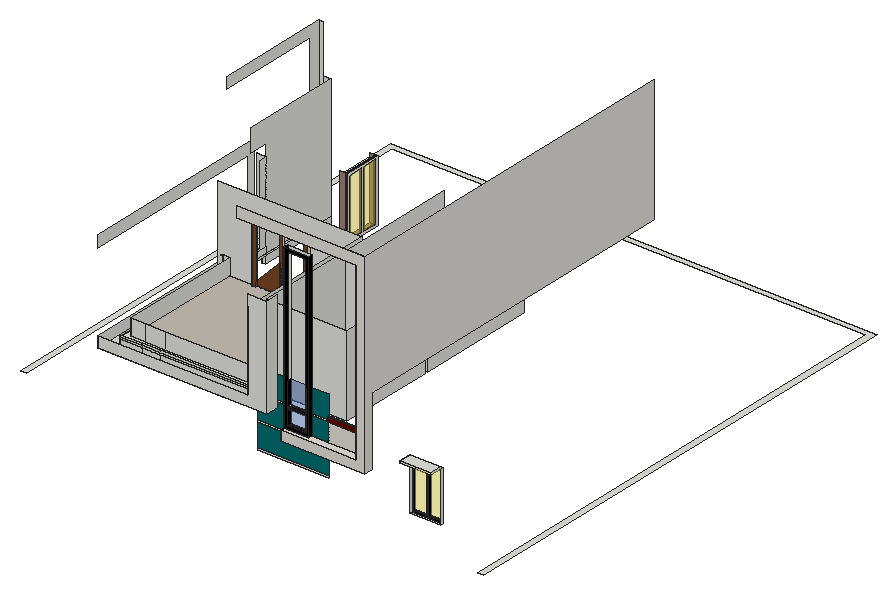
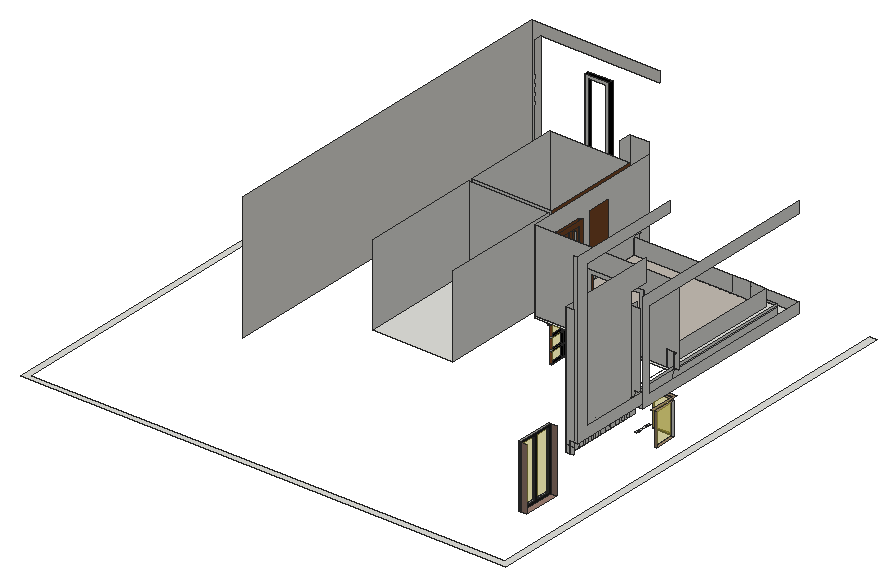
# SketchUp Ruby script. Lengths in inches.
U = 1.inch
M = Sketchup.active_model
def pt(a) = Geom::Point3d.new(a.map { |v| v * U })
def face(e, loops, mat)
  f = e.add_face(loops[0].map { |a| pt(a) })
  loops[1..].each { |l| e.add_face(l.map { |a| pt(a) }).erase! }
  f.material = f.back_material = mat if mat
  f
end
# faces: each face lists its corners as indices into pts; further lists are holes
def faces(e, pts, list, mat = nil) = list.each { |f| face(e, (f[0].is_a?(Array) ? f : [f]).map { |l| l.map { |i| pts[i] } }, mat) }
# xy, xz, yz: faces in a plane at the given z, y or x. An outline is a flat list of corners, or four numbers for a rectangle; further outlines are holes
def ring(l) = l.size == 4 ? [[l[0], l[1]], [l[2], l[1]], [l[2], l[3]], [l[0], l[3]]] : l.each_slice(2).to_a
def flat(e, list, mat, &to3) = list.each { |f| face(e, (f[0].is_a?(Array) ? f : [f]).map { |l| ring(l).map { |u, v| to3.(u, v) } }, mat) }
def xy(e, z, list, mat = nil) = flat(e, list, mat) { |x, y| [x, y, z] }
def xz(e, y, list, mat = nil) = flat(e, list, mat) { |x, z| [x, y, z] }
def yz(e, x, list, mat = nil) = flat(e, list, mat) { |y, z| [x, y, z] }
def lines(e, pts, list) = list.each { |a, b| e.add_line(pt(pts[a]), pt(pts[b])) }
# prism: a flat outline (further loops are holes) pulled along v
def prism(e, loops, v, mat = nil)
  f = face(e, loops, mat); d = Geom::Vector3d.new(v.map { |x| x * U })
  f.pushpull(f.normal.samedirection?(d) ? d.length : -d.length)
end
def box(e, o, s, mat = nil) = prism(e, [[o, [o[0] + s[0], o[1], o[2]], [o[0] + s[0], o[1] + s[1], o[2]], [o[0], o[1] + s[1], o[2]]]], [0, 0, s[2]], mat)
def at(x, y, z, deg = 0) = Geom::Transformation.translation(pt([x, y, z])) * Geom::Transformation.rotation(ORIGIN, Z_AXIS, deg.degrees)
def axes(o, x, y, z) = Geom::Transformation.new([*x, 0, *y, 0, *z, 0, *pt(o).to_a, 1])
def part(name) = M.definitions.add(name)
# library, detail: a bought-in or finely detailed component or shape, given as its bounding box
def library(name, o, s) = part(name).tap { |d| box(d.entities, o, s) }
def detail(e, o, s) = box(e.add_group.entities, o, s)
def put(e, d, t, mat = nil) = e.add_instance(d, t).tap { |i| i.material = mat if mat }
def group(e, t, mat = nil) = e.add_group.tap { |g| g.transformation = t; g.material = mat if mat }.entities
root = M.entities
M.materials.add("Niraj_Skin").color = [158, 128, 115]
M.materials.add("[0035_Tan]").color = [158, 135, 105]
M.materials.add("[Color A08]").color = [102, 0, 0]
M.materials.add("[Color H07]1").color = [0, 109, 109]
M.materials.add("[Color M08]").color = [30, 30, 30]
M.materials.add("[Color M09]").color = [0, 0, 0]
M.materials.add("[Field Rectangle Tile]").color = [196, 189, 179]
M.materials.add("[Marble Carrara Gold Floor Tile]").color = [225, 223, 217]
M.materials.add("[Translucent Glass Blue]1").color = [78, 117, 186]
M.materials["[Translucent Glass Blue]1"].alpha = 0.5
M.materials.add("[Translucent Glass Gray]").color = [242, 225, 74]
M.materials["[Translucent Glass Gray]"].alpha = 0.5
M.materials.add("[Wood Cherry Original]").color = [152, 86, 42]
M.materials.add("[Wood Veneer 01]").color = [120, 70, 37]
xy(root,45.05,[[92.54,302.6,119.85,305.6]],"[0035_Tan]")
xy(root,45.39,[[86.54,308.6,89.54,339.85]],"[0035_Tan]")
xy(root,53.97,[[524.95,106.91,571.13,109.91]])
xy(root,56.97,[[527.95,109.91,548.04,112.91],[550.83,109.91,568.13,112.91]],"[Color M09]")
xy(root,58.26,[[288.79,233.45,291.79,257.5625],[288.79,260.11,291.79,280.89]],"[Color M09]")
xy(root,60.09,[[288.79,233.45,291.79,257.5625],[288.79,260.11,291.79,280.89]],"[Color M09]")
xy(root,70,[[86.54,536.21,89.54,591.21]])
xy(root,70,[[77.54,536.21,86.54,591.21]],"Niraj_Skin")
xy(root,73,[[86.54,539.21,89.54,562],[86.54,565,89.54,588.21]],"[Color M08]")
xy(root,75.82,[[288.79,233.45,291.79,257.5625],[288.79,260.11,291.79,280.89]],"[Color M09]")
xy(root,77.65,[[288.79,233.45,291.79,257.5625],[288.79,260.11,291.79,280.89]],"[Color M09]")
xy(root,80.4,[[86.54,350.68,89.54,354.7],[86.54,357.49,89.54,361.52],[86.54,364.68,89.54,368.7],[86.54,371.93,89.54,375.95]])
xy(root,86.53,[[338.5625,100.91,463.41,112.91]])
xy(root,87.61,[[711.33,0,720.33,0,720.33,727.14,0,727.14,0,40.8125,9,40.8125,9,718.14,711.33,718.14]])
xy(root,92.95,[[92.54,302.6,119.85,305.6],[86.54,308.6,89.54,339.85]],"[0035_Tan]")
xy(root,93.38,[[288.79,233.45,291.79,257.5625],[288.79,260.11,291.79,280.89]],"[Color M09]")
xy(root,95.22,[[288.79,233.45,291.79,257.5625],[288.79,260.11,291.79,280.89]],"[Color M09]")
xy(root,97.01,[[86.54,302.6,123.91,302.6,123.91,305.6,89.54,305.6,89.54,346.85,86.54,346.85]],"[0035_Tan]")
xy(root,100.57,[[291.79,136.74,294.79,157.71],[291.79,160.71,294.79,184.67]],"[Color M09]")
xy(root,101.25,[[338.5625,100.91,449.03,100.91,449.03,112.91,374.46,112.91,374.46,106.91,338.5625,106.91]],"[Marble Carrara Gold Floor Tile]")
xy(root,105.75,[[291.79,131.57,294.79,189.85]])
xy(root,105.77,[[343.08,106.91,369.95,112.91]],"[Color M09]")
xy(root,109.36,[[291.79,233.45,294.79,280.89],[288.79,257.5625,291.79,260.11],[288.79,260.11,291.79,280.89]])
xy(root,109.36,[[288.79,233.45,291.79,257.5625]],"[Wood Cherry Original]")
xy(root,110.36,[[84.04,383.99,89.54,504.04]])
xy(root,115.36,[[288.79,227.45,294.79,286.89]],"[Wood Cherry Original]")
xy(root,120.61,[[72.04,94.04,72.04,383.99,89.54,383.99,89.54,112.91,322.48,112.91,322.48,94.04]])
xy(root,125.66,[[527.95,109.91,548.04,112.91],[550.83,109.91,568.13,112.91]],"[Color M09]")
xy(root,127.49,[[72.04,383.99,72.04,504.04,84.04,504.04,84.04,503.21,81.04,503.21,81.04,496.61,84.04,496.61,84.04,494.46,81.04,494.46,81.04,487.86,84.04,487.86,84.04,484.77,81.04,484.77,81.04,478.18,84.04,478.18,84.04,475.21,81.04,475.21,81.04,468.61,84.04,468.61,84.04,465.65,81.04,465.65,81.04,459.05,84.04,459.05,84.04,456.09,81.04,456.09,81.04,449.49,84.04,449.49,84.04,446.52,81.04,446.52,81.04,439.93,84.04,439.93,84.04,436.96,81.04,436.96,81.04,430.36,84.04,430.36,84.04,427.4,81.04,427.4,81.04,420.8,84.04,420.8,84.04,417.84,81.04,417.84,81.04,411.24,84.04,411.24,84.04,408.27,81.04,408.27,81.04,401.68,84.04,401.68,84.04,398.71,81.04,398.71,81.04,392.11,84.04,392.11,84.04,383.99],[81.04,392.11,84.04,398.71],[81.04,401.68,84.04,408.27],[81.04,411.24,84.04,417.84],[81.04,420.8,84.04,427.4],
  [81.04,430.36,84.04,436.96],[81.04,439.93,84.04,446.52],[81.04,449.49,84.04,456.09],[81.04,459.05,84.04,465.65],[81.04,468.61,84.04,475.21],
  [81.04,478.18,84.04,484.77],[81.04,487.86,84.04,494.46],[81.04,496.61,84.04,503.21]])
xy(root,128.34,[[343.08,106.91,369.95,112.91]],"[Color M09]")
xy(root,128.66,[[524.95,88.04,571.13,109.91],[571.13,88.04,571.26,106.91]])
xy(root,129.61,[[89.54,112.91,294.79,305.6]])
xy(root,129.75,[[400.27,109.91,449.03,112.91]],"[Color A08]")
xy(root,130.72,[[343.08,106.91,369.95,112.91]],"[Color M09]")
xy(root,131.79,[[524.95,88.04,571.26,106.91]])
xy(root,132.61,[[89.54,112.91,89.54,305.6,98.54,305.6,98.54,121.91,294.79,121.91,294.79,112.91],[294.79,121.91,300.66,266.1],[300.66,121.91,300.79,266.1],[300.79,121.91,419.79,266.1],[288.79,223.6,294.79,229.6],
  [291.79,229.6,294.79,229.6,294.79,266.1,291.79,266.1,291.79,247.85,288.79,247.85,288.79,243.65,291.79,243.65],[288.79,266.1,294.79,272.1],[300.79,272.1,419.79,449.91],[133.47,302.6,139.47,305.6],[175.47,302.6,178.47,305.6],
  [195.5,302.6,199.42,305.6],[203.33,302.6,207.24,305.6],[211.16,302.6,211.47,305.6],[211.47,302.6,217.47,305.6]])
xy(root,132.61,[[98.54,121.91,294.79,121.91,294.79,223.6,288.79,223.6,288.79,229.6,291.79,229.6,291.79,243.65,288.79,243.65,288.79,247.85,291.79,247.85,291.79,266.1,288.79,266.1,288.79,272.1,294.79,272.1,294.79,305.6,217.47,305.6,217.47,302.6,211.16,302.6,211.16,305.6,207.24,305.6,207.24,302.6,203.33,302.6,203.33,305.6,199.42,305.6,199.42,302.6,195.5,302.6,195.5,305.6,178.47,305.6,178.47,302.6,175.47,302.6,175.47,305.6,139.47,305.6,139.47,302.6,133.47,302.6,133.47,305.6,98.54,305.6]],"[Field Rectangle Tile]")
xz(root,88.04,[[524.95,128.66,571.26,131.79]])
xz(root,94.04,[[72.04,120.61,322.48,120.61,322.48,269.74,294.79,269.74,294.79,135.72,72.04,135.72]])
xz(root,100.91,[[338.5625,86.53,463.41,86.53,463.41,375.61,272.85,375.61,272.85,359.87,449.03,359.87,449.03,101.25,338.5625,101.25]],"[Marble Carrara Gold Floor Tile]")
xz(root,106.91,[[[338.5625,101.25,374.46,341.53],[343.08,105.77,369.95,337.01]],[343.08,128.34,369.95,130.72]],"[Color M09]")
xz(root,109.91,[[400.27,129.75,449.03,136.63]],"[Color A08]")
xz(root,109.91,[[[524.95,53.97,571.13,128.66],[527.95,56.97,548.04,125.66],[550.83,56.97,568.13,125.66]]],"[Color M09]")
xz(root,112.91,[[294.79,54.34,400.27,56.72],[338.5625,86.53,400.27,91.34],[294.79,91.34,338.5625,93.72],[338.5625,91.34,400.27,93.72],[338.5625,93.72,400.27,101.25],
  [[338.5625,101.25,374.46,341.53],[343.08,105.77,369.95,337.01]],[89.54,120.61,121.875,129.61],[121.875,120.61,149.09,129.61],[149.09,120.61,294.79,129.61],[294.79,120.61,322.48,128.34],
  [294.79,128.34,322.48,130.72],[322.48,128.34,338.5625,130.72],[343.08,128.34,369.95,130.72],[374.46,128.34,400.27,130.72],[89.54,129.61,121.875,132.61],
  [121.875,129.61,149.09,132.61],[149.09,129.61,294.79,132.61],[400.27,129.75,449.03,136.63],[294.79,130.72,322.48,132.61],[89.54,132.61,121.875,135.72],
  [121.875,132.61,149.09,135.72],[149.09,132.61,294.79,135.72],[294.79,132.61,322.48,165.34]])
xz(root,112.91,[[294.79,56.72,400.27,56.72,400.27,86.53,338.5625,86.53,338.5625,91.34,294.79,91.34],[294.79,93.72,338.5625,93.72,338.5625,128.34,322.48,128.34,322.48,120.61,294.79,120.61],[374.46,101.25,400.27,128.34],[322.48,130.72,338.5625,165.34],[374.46,130.72,400.27,165.34]],"[Color H07]1")
xz(root,112.91,[[400.27,101.25,449.03,129.75]],"[Marble Carrara Gold Floor Tile]")
xz(root,112.91,[[343.08,105.77,369.95,128.34],[343.08,130.72,369.95,165.34]],"[Translucent Glass Blue]1")
xz(root,112.91,[[527.95,56.97,548.04,125.66],[550.83,56.97,568.13,125.66]],"[Translucent Glass Gray]")
xz(root,121.91,[[98.54,132.61,121.875,156.61],[121.875,132.61,149.09,156.61],[149.09,132.61,294.79,156.61],[300.66,132.61,300.79,252.61],[300.79,132.61,419.79,252.61]])
xz(root,223.6,[[288.79,132.61,294.79,226.55]],"[Wood Veneer 01]")
xz(root,229.6,[[291.79,132.61,294.79,220.55]])
xz(root,229.6,[[288.79,132.61,291.79,220.55]],"[Wood Veneer 01]")
xz(root,233.45,[[288.79,58.26,291.79,60.09],[288.79,75.82,291.79,77.65],[288.79,93.38,291.79,95.22]])
xz(root,233.45,[[288.79,60.09,291.79,75.82],[288.79,77.65,291.79,93.38],[288.79,95.22,291.79,109.36]],"[Wood Cherry Original]")
xz(root,243.65,[[288.79,132.61,291.79,220.55]],"[Wood Veneer 01]")
xz(root,247.85,[[288.79,132.61,291.79,220.55]],"[Wood Veneer 01]")
xz(root,257.5625,[[288.79,60.09,291.79,75.82],[288.79,77.65,291.79,93.38],[288.79,95.22,291.79,109.36]],"[Color M09]")
xz(root,260.11,[[288.79,60.09,291.79,75.82],[288.79,77.65,291.79,93.38],[288.79,95.22,291.79,109.36]],"[Color M09]")
xz(root,266.1,[[291.79,132.61,294.79,220.55],[300.66,132.61,300.79,252.61],[300.79,132.61,419.79,252.61]])
xz(root,266.1,[[288.79,132.61,291.79,220.55]],"[Wood Veneer 01]")
xz(root,272.1,[[300.79,132.61,419.79,252.61]])
xz(root,272.1,[[288.79,132.61,294.79,226.55]],"[Wood Veneer 01]")
xz(root,280.89,[[288.79,58.26,291.79,60.09],[288.79,75.82,291.79,77.65],[288.79,93.38,291.79,95.22]])
xz(root,280.89,[[288.79,60.09,291.79,75.82],[288.79,77.65,291.79,93.38],[288.79,95.22,291.79,109.36]],"[Wood Cherry Original]")
xz(root,302.6,[[133.47,132.61,139.47,132.61,139.47,216.61,175.47,216.61,175.47,132.61,178.47,132.61,178.47,216.61,211.47,216.61,211.47,132.61,217.47,132.61,217.47,222.61,133.47,222.61],[195.5,132.61,199.42,132.61,178.47,154.69,178.47,150.57],[203.33,132.61,207.24,132.61,178.47,162.94,178.47,158.82],[211.16,132.61,211.47,132.61,211.47,136.41,178.47,171.19,178.47,167.07]],"[Wood Veneer 01]")
xz(root,305.6,[[133.47,129.61,198.35,129.61,195.5,132.61,133.47,132.61],[198.35,129.61,202.26,129.61,199.42,132.61,195.5,132.61],[202.26,129.61,206.18,129.61,203.33,132.61,199.42,132.61],[206.18,129.61,210.09,129.61,207.24,132.61,203.33,132.61],[210.09,129.61,217.47,129.61,217.47,132.61,207.24,132.61],
  [98.54,132.61,133.47,132.61,133.47,222.61,217.47,222.61,217.47,132.61,294.79,132.61,294.79,252.61,80.6,252.61,80.6,135.72,86.54,135.72,86.54,154.35,83.54,154.35,83.54,156.61,98.54,156.61],[89.54,132.61,98.54,156.61],[133.47,132.61,133.47,222.61,217.47,222.61,217.47,132.61,211.47,132.61,211.47,216.61,178.47,216.61,178.47,132.61,175.47,132.61,175.47,216.61,139.47,216.61,139.47,132.61],[195.5,132.61,178.47,150.57,178.47,154.69,199.42,132.61],[203.33,132.61,178.47,158.82,178.47,162.94,207.24,132.61],
  [211.16,132.61,178.47,167.07,178.47,171.19,211.47,136.41,211.47,132.61]])
xz(root,305.6,[[92.54,45.05,119.85,92.95]],"[Translucent Glass Gray]")
xz(root,305.6,[[139.47,132.61,175.47,132.61,175.47,178,139.47,139.77],[178.47,132.61,195.5,132.61,178.47,150.57],[199.42,132.61,203.33,132.61,178.47,158.82,178.47,154.69],[207.24,132.61,211.16,132.61,178.47,167.07,178.47,162.94]],"[Wood Veneer 01]")
xz(root,308.6,[[86.54,45.39,89.54,92.95]])
xz(root,339.85,[[86.54,45.39,89.54,92.95]],"[0035_Tan]")
xz(root,383.99,[[84.04,110.36,89.54,120.61],[72.04,120.61,84.04,127.49],[84.04,120.61,89.54,132.61],[72.04,127.49,84.04,132.61],[72.04,132.61,72.04,143.24,76.23,143.24,76.23,140.99,84.04,140.99,84.04,132.61],
  [84.04,132.61,84.04,140.99,76.23,140.99,76.23,252.61,89.54,252.61,89.54,132.61]])
xz(root,504.04,[[77.54,110.36,84.04,120.61],[84.04,110.36,89.54,120.61],[77.54,120.61,84.04,127.49],[84.04,120.61,84.04,127.49,77.54,127.49,77.54,303.61,89.54,303.61,89.54,120.61],[72.04,127.49,77.54,375.61]])
xz(root,536.21,[[86.54,70,89.54,162.875]])
xz(root,536.21,[[77.54,70,86.54,162.875]],"Niraj_Skin")
xz(root,539.21,[[86.54,73,89.54,159.875]],"[Color M08]")
xz(root,562,[[86.54,73,89.54,159.875]],"[Color M08]")
xz(root,565,[[86.54,73,89.54,159.875]],"[Color M08]")
xz(root,588.21,[[86.54,73,89.54,159.875]],"[Color M08]")
xz(root,591.21,[[86.54,70,89.54,162.875]])
xz(root,591.21,[[77.54,70,86.54,162.875]],"Niraj_Skin")
yz(root,72.04,[[94.04,120.61,94.04,135.72,372.52,135.72,372.52,252.61,94.04,252.61,94.04,269.74,383.99,269.74,383.99,120.61],[383.99,127.49,383.99,143.24,487.33,143.24,487.33,359.2,332.99,359.2,332.99,375.61,504.04,375.61,504.04,127.49]])
yz(root,84.04,[[383.99,110.36,392.11,127.49],[392.11,110.36,398.71,127.49],[398.71,110.36,401.68,127.49],[401.68,110.36,408.27,127.49],[408.27,110.36,411.24,127.49],
  [411.24,110.36,417.84,127.49],[417.84,110.36,420.8,127.49],[420.8,110.36,427.4,127.49],[427.4,110.36,430.36,127.49],[430.36,110.36,436.96,127.49],
  [436.96,110.36,439.93,127.49],[439.93,110.36,446.52,127.49],[446.52,110.36,449.49,127.49],[449.49,110.36,456.09,127.49],[456.09,110.36,459.05,127.49],
  [459.05,110.36,465.65,127.49],[465.65,110.36,468.61,127.49],[468.61,110.36,475.21,127.49],[475.21,110.36,478.18,127.49],[478.18,110.36,484.77,127.49],
  [484.77,110.36,487.86,127.49],[487.86,110.36,494.46,127.49],[494.46,110.36,496.61,127.49],[496.61,110.36,503.21,127.49],[503.21,110.36,504.04,127.49]])
yz(root,86.54,[[[536.21,70,591.21,162.875],[565,73,588.21,159.875],[539.21,73,562,159.875]]],"[Color M08]")
yz(root,89.54,[[[536.21,70,591.21,162.875],[565,73,588.21,159.875],[539.21,73,562,159.875]],[383.99,110.36,504.04,120.61],[112.91,120.61,305.6,129.61],[305.6,120.61,305.6,129.61,112.91,129.61,112.91,132.61,383.99,132.61,383.99,120.61],[383.99,120.61,504.04,120.61,504.04,303.61,355.8,303.61,355.8,269.74,383.99,269.74],
  [112.91,132.61,305.6,135.72],[305.6,132.61,383.99,132.61,383.99,252.61,372.52,252.61,372.52,135.72,305.6,135.72]])
yz(root,89.54,[[308.6,45.39,339.85,92.95],[539.21,73,562,159.875],[565,73,588.21,159.875]],"[Translucent Glass Gray]")
yz(root,92.54,[[302.6,45.05,305.6,92.95]],"[0035_Tan]")
yz(root,98.54,[[121.91,132.61,305.6,156.61]])
yz(root,119.85,[[302.6,45.05,305.6,92.95]],"[0035_Tan]")
yz(root,133.47,[[302.6,132.61,305.6,222.61]],"[Wood Veneer 01]")
yz(root,139.47,[[302.6,132.61,305.6,139.77]],"[Wood Veneer 01]")
yz(root,175.47,[[302.6,132.61,305.6,178]],"[Wood Veneer 01]")
yz(root,178.47,[[302.6,132.61,305.6,150.57]],"[Wood Veneer 01]")
yz(root,211.47,[[302.6,132.61,305.6,136.41]])
yz(root,217.47,[[302.6,132.61,305.6,222.61]])
yz(root,288.79,[[223.6,132.61,223.6,226.55,272.1,226.55,272.1,132.61,266.1,132.61,266.1,220.55,229.6,220.55,229.6,132.61],[243.65,132.61,247.85,220.55]],"[Wood Veneer 01]")
yz(root,291.79,[[233.45,60.09,257.5625,75.82],[260.11,60.09,280.89,75.82],[233.45,77.65,257.5625,93.38],[260.11,77.65,280.89,93.38],[233.45,95.22,257.5625,109.36],
  [260.11,95.22,280.89,109.36]],"[Translucent Glass Gray]")
yz(root,291.79,[[[229.6,132.61,243.65,220.55],[236.45,186.16,237.5,186.28,238.5,186.65,239.39,187.23,240.11,188,240.65,188.91,240.95,189.93,240.95,213.28,240.57,214.21,240,215.04,239.27,215.72,238.4,216.24,237.45,216.55,236.45,216.66,235.45,216.55,234.5,216.24,233.64,215.72,232.9,215.04,232.33,214.21,231.95,213.28,231.95,189.93,232.26,188.91,232.79,188,233.52,187.23,234.4,186.65,235.4,186.28],[236.45,141.38,237.62,141.54,238.7,141.99,239.63,142.7,240.35,143.63,240.8,144.72,240.95,145.88,240.95,167.68,240.73,168.78,240.24,169.79,239.52,170.65,238.61,171.3,237.57,171.71,236.45,171.85,235.34,171.71,234.3,171.3,233.39,170.65,232.66,169.79,232.18,168.78,231.95,167.68,231.95,145.88,232.11,144.72,232.56,143.63,233.27,142.7,234.2,141.99,235.29,141.54]],[[247.85,132.61,266.1,220.55],[257.39,141.35,258.51,141.49,259.56,141.9,260.47,142.5625,261.19,143.43,261.67,144.45,261.89,145.55,261.89,167.31,261.74,168.47,261.29,169.56,260.57,170.49,259.64,171.21,258.55,171.65,257.39,171.81,256.23,171.65,255.14,171.21,254.21,170.49,253.49,169.56,253.04,168.47,252.89,167.31,252.89,145.55,253.11,144.45,253.59,143.43,254.3125,142.5625,255.22,141.9,256.27,141.49],[256.39,186.3,257.55,186.45,258.64,186.9,259.57,187.61,260.29,188.55,260.74,189.63,260.89,190.8,260.89,213.15,260.53,214.11,259.98,214.97,259.24,215.68,258.375,216.22,257.41,216.55,256.39,216.66,255.375,216.55,254.41,216.22,253.54,215.68,252.8,214.97,252.25,214.11,251.89,213.15,251.89,190.8,252.04,189.63,252.49,188.55,253.21,187.61,254.14,186.9,255.23,186.45]]],"[Wood Veneer 01]")
yz(root,294.79,[[112.91,129.61,121.91,132.61],[121.91,129.61,266.1,132.61],[266.1,129.61,272.1,132.61],[[121.91,132.61,121.91,156.61,106.91,156.61,106.91,154.35,109.91,154.35,109.91,135.72,94.04,135.72,94.04,252.61,305.6,252.61,305.6,132.61,272.1,132.61,272.1,226.55,223.6,226.55,223.6,132.61],[167.29,165.31,205.98,227.91]],[112.91,132.61,121.91,156.61],
  [[229.6,132.61,266.1,220.55],[236.45,186.16,237.5,186.28,238.5,186.65,239.39,187.23,240.11,188,240.65,188.91,240.95,189.93,240.95,213.28,240.57,214.21,240,215.04,239.27,215.72,238.4,216.24,237.45,216.55,236.45,216.66,235.45,216.55,234.5,216.24,233.64,215.72,232.9,215.04,232.33,214.21,231.95,213.28,231.95,189.93,232.26,188.91,232.79,188,233.52,187.23,234.4,186.65,235.4,186.28],[236.45,141.38,237.62,141.54,238.7,141.99,239.63,142.7,240.35,143.63,240.8,144.72,240.95,145.88,240.95,167.68,240.73,168.78,240.24,169.79,239.52,170.65,238.61,171.3,237.57,171.71,236.45,171.85,235.34,171.71,234.3,171.3,233.39,170.65,232.66,169.79,232.18,168.78,231.95,167.68,231.95,145.88,232.11,144.72,232.56,143.63,233.27,142.7,234.2,141.99,235.29,141.54],[257.39,141.35,258.51,141.49,259.56,141.9,260.47,142.5625,261.19,143.43,261.67,144.45,261.89,145.55,261.89,167.31,261.74,168.47,261.29,169.56,260.57,170.49,259.64,171.21,258.55,171.65,257.39,171.81,256.23,171.65,255.14,171.21,254.21,170.49,253.49,169.56,253.04,168.47,252.89,167.31,252.89,145.55,253.11,144.45,253.59,143.43,254.3125,142.5625,255.22,141.9,256.27,141.49],[256.39,186.3,257.55,186.45,258.64,186.9,259.57,187.61,260.29,188.55,260.74,189.63,260.89,190.8,260.89,213.15,260.53,214.11,259.98,214.97,259.24,215.68,258.375,216.22,257.41,216.55,256.39,216.66,255.375,216.55,254.41,216.22,253.54,215.68,252.8,214.97,252.25,214.11,251.89,213.15,251.89,190.8,252.04,189.63,252.49,188.55,253.21,187.61,254.14,186.9,255.23,186.45]],[266.1,132.61,272.1,226.55]])
yz(root,300.66,[[121.91,132.61,266.1,252.61]],"[Wood Veneer 01]")
yz(root,300.79,[[121.91,132.61,266.1,252.61],[272.1,132.61,449.91,252.61]])
yz(root,322.48,[[94.04,120.61,112.91,269.74]])
yz(root,338.5625,[[100.91,86.53,100.91,101.25,106.91,101.25,106.91,341.53,112.91,341.53,112.91,86.53]],"[Color M09]")
yz(root,343.08,[[106.91,128.34,112.91,130.72]])
yz(root,343.08,[[106.91,105.77,112.91,128.34],[106.91,130.72,112.91,165.34]],"[Color M09]")
yz(root,369.95,[[106.91,105.77,112.91,128.34],[106.91,130.72,112.91,165.34]],"[Color M09]")
yz(root,374.46,[[106.91,101.25,112.91,341.53]],"[Color M09]")
yz(root,400.27,[[109.91,129.75,112.91,136.63]],"[Color A08]")
yz(root,419.79,[[121.91,132.61,266.1,252.61],[272.1,132.61,449.91,252.61]])
yz(root,449.03,[[109.91,129.75,112.91,136.63]])
yz(root,449.03,[[100.91,101.25,100.91,359.87,112.91,359.87,112.91,314.2,109.91,314.2,109.91,307.31,112.91,307.31,112.91,303.01,109.91,303.01,109.91,296.12,112.91,296.12,112.91,290.7,109.91,290.7,109.91,283.81,112.91,283.81,112.91,278.95,109.91,278.95,109.91,272.06,112.91,272.06,112.91,170.51,109.91,170.51,109.91,163.62,112.91,163.62,112.91,159.01,109.91,159.01,109.91,152.12,112.91,152.12,112.91,147.57,109.91,147.57,109.91,140.68,112.91,140.68,112.91,136.63,109.91,136.63,109.91,129.75,112.91,129.75,112.91,101.25]],"[Marble Carrara Gold Floor Tile]")
yz(root,463.41,[[100.91,86.53,112.91,86.53,112.91,188.93,636.48,188.93,636.48,375.61,100.91,375.61]],"[Marble Carrara Gold Floor Tile]")
yz(root,524.95,[[106.91,53.97,109.91,128.66],[88.04,128.66,106.91,131.79]])
yz(root,527.95,[[109.91,56.97,112.91,125.66]],"[Color M09]")
yz(root,548.04,[[109.91,56.97,112.91,125.66]],"[Color M09]")
yz(root,550.83,[[109.91,56.97,112.91,125.66]],"[Color M09]")
yz(root,568.13,[[109.91,56.97,112.91,125.66]],"[Color M09]")
yz(root,571.13,[[106.91,53.97,109.91,128.66]])
yz(root,571.26,[[88.04,128.66,106.91,131.79]])
p = [[178.47,305.6,167.07],[211.16,305.6,132.61],[211.16,302.6,132.61],[178.47,302.6,167.07],[178.47,305.6,158.82],[203.33,305.6,132.61],
  [203.33,302.6,132.61],[178.47,302.6,158.82],[207.24,305.6,132.61],[178.47,305.6,162.94],[178.47,302.6,162.94],[207.24,302.6,132.61],
  [178.47,305.6,150.57],[195.5,305.6,132.61],[195.5,302.6,132.61],[178.47,302.6,150.57],[199.42,305.6,132.61],[178.47,305.6,154.69],
  [178.47,302.6,154.69],[199.42,302.6,132.61],[98.54,305.6,132.61],[98.54,449.91,132.61],[89.54,449.91,132.61],[211.47,305.6,132.28]]
faces(root,p,[[0,1,2,3],[4,5,6,7],[8,9,10,11],[12,13,14,15],[16,17,18,19]],"[Wood Veneer 01]")
lines(root,p,[[20,21],[21,22],[1,23]])
